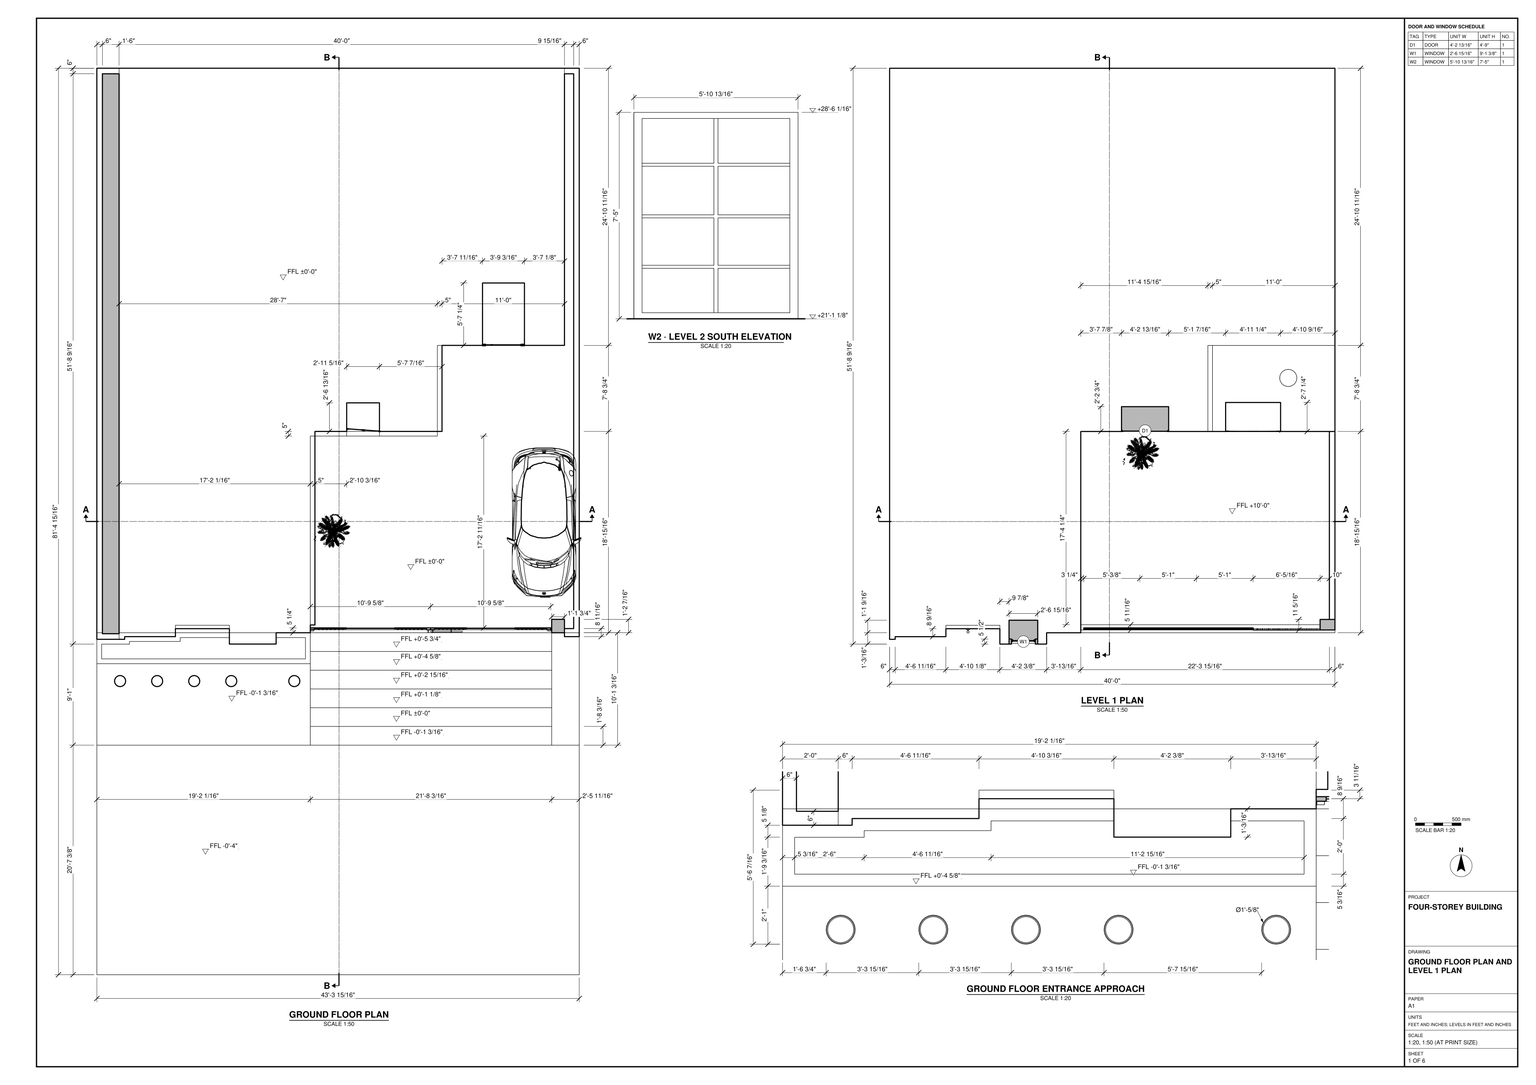
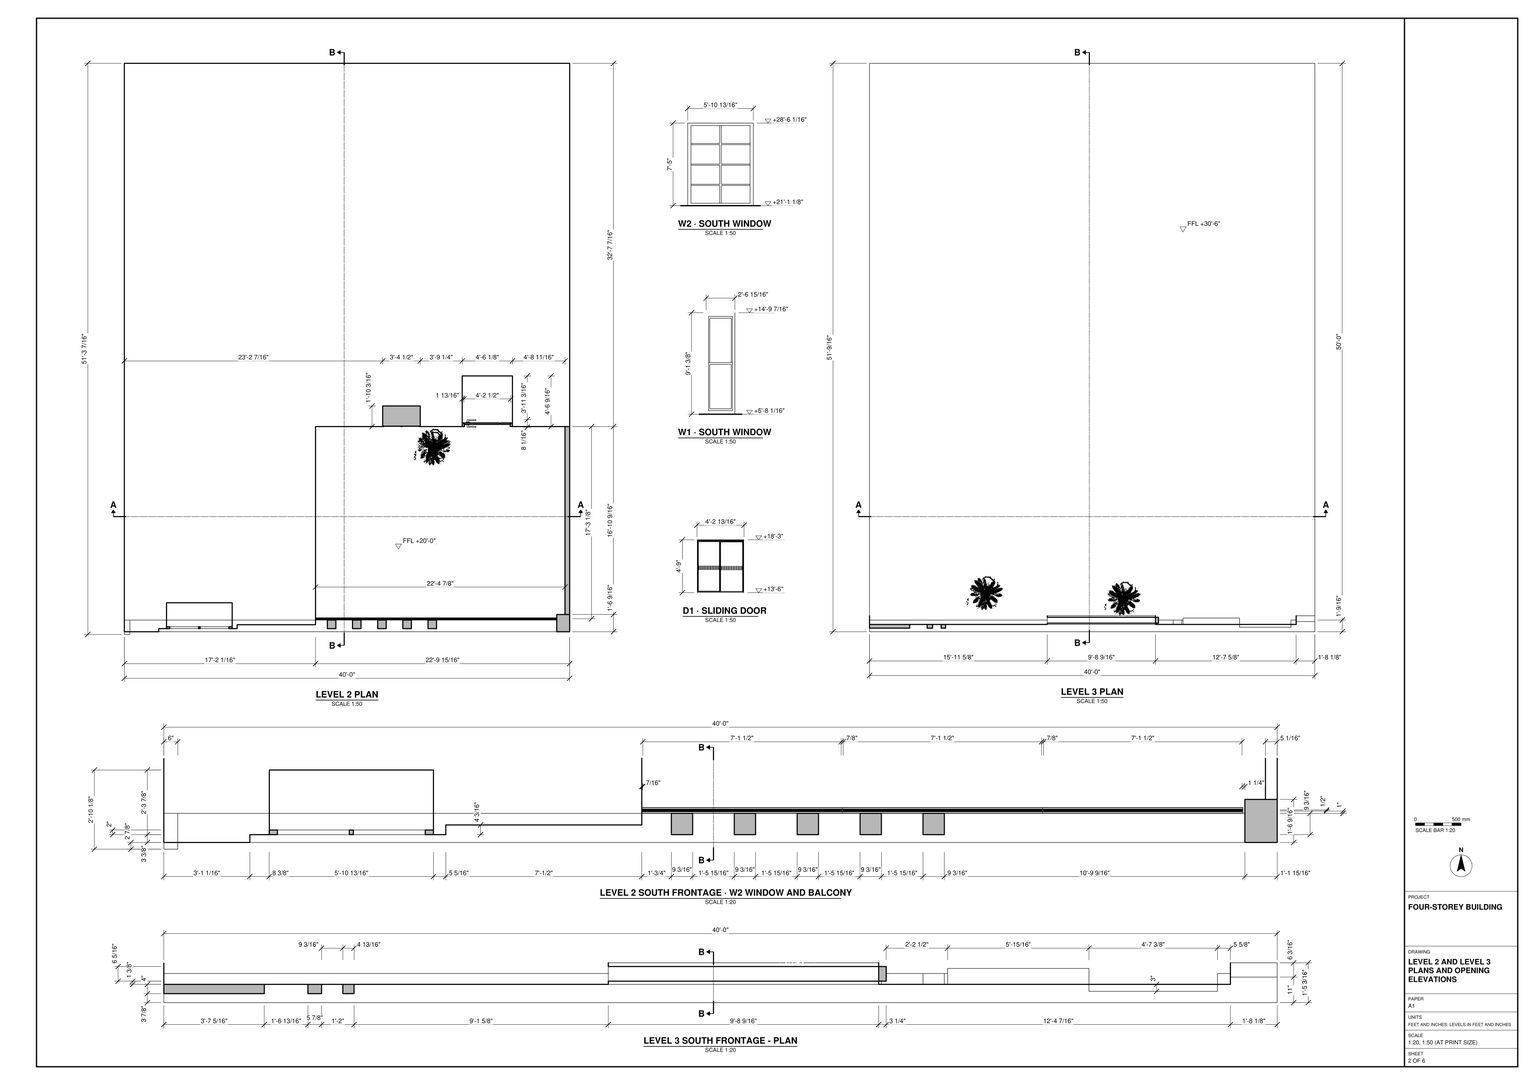
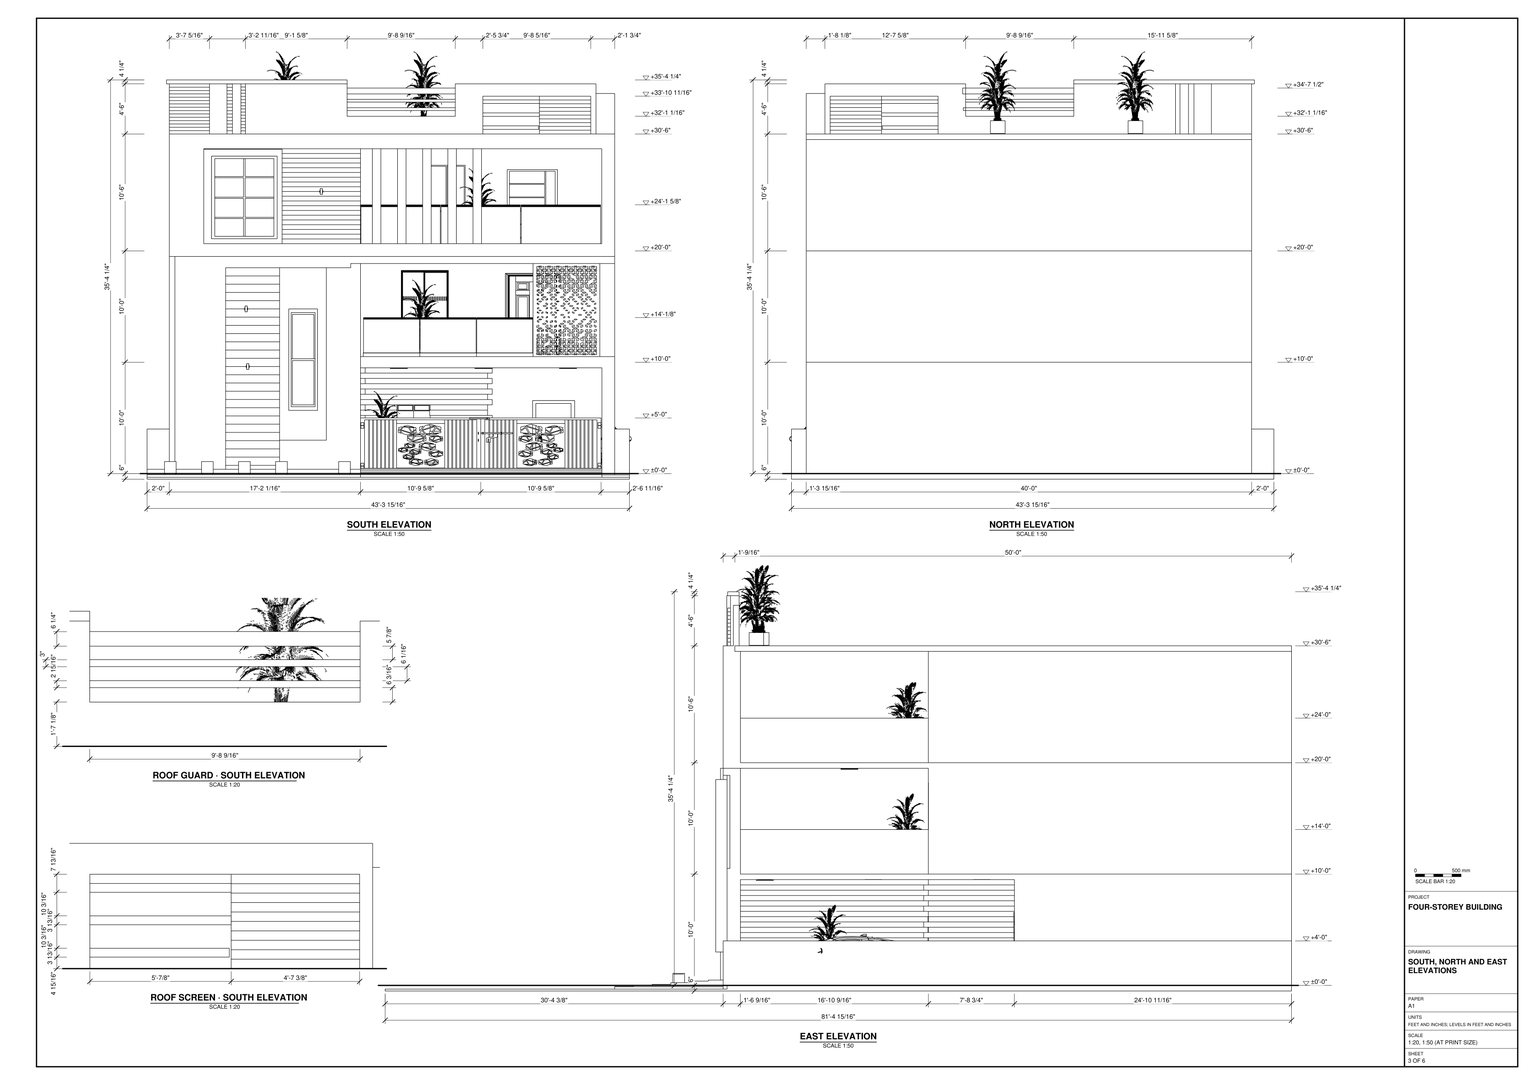
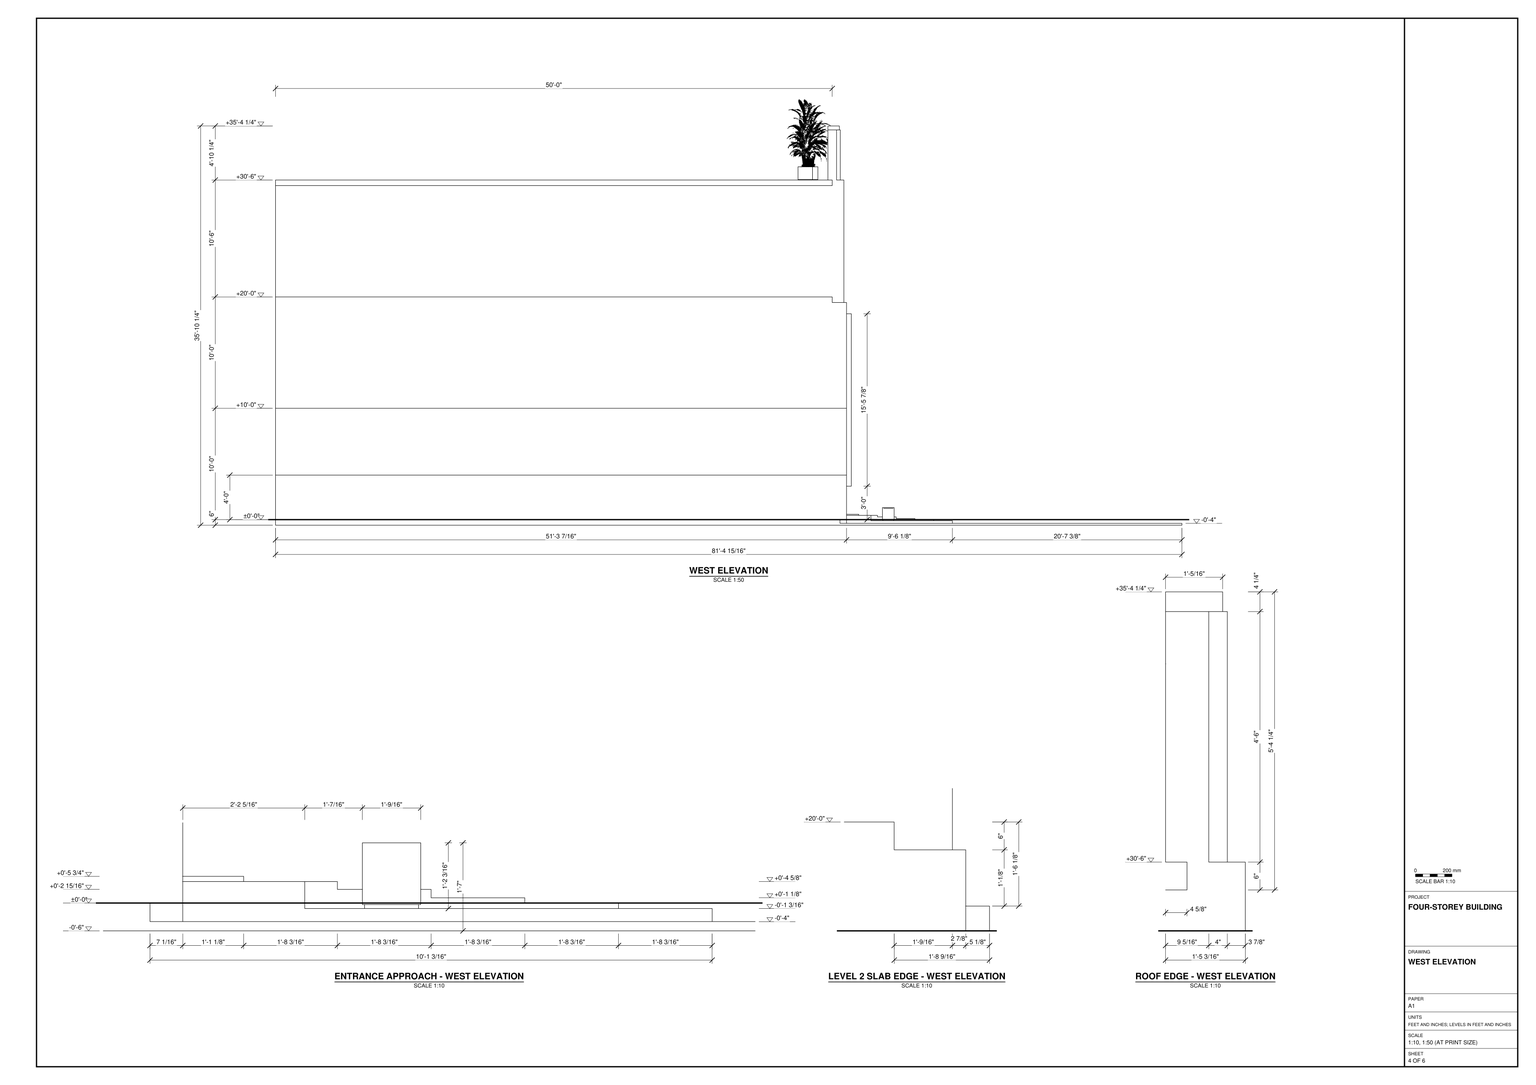
Use task_files/diagram_01.pdf to build the building and its south entrance approach in SketchUp. Work in feet and inches. Including the approach and roof planting, the overall model extents are 43'-5 15/16" across the frontage, 81'-4 15/16" from front to back and 38'-5 9/16" in height. Set the ground floor at ±0'-0", Level 1 at +10'-0", Level 2 at +20'-0" and the roof terrace at +30'-6".

Follow the plans for the wall thicknesses, slab edges and changes in footprint. Set the covered parking bay behind the paired entrance gate on the right when viewed from the south. Model the shallow changes of level across the approach and the two recessed balconies above the bay. Use the opening details for the sliding door, the tall narrow window and the wider divided window. Match the south elevation's projecting window surround, horizontal bands, vertical fins, balcony guards and patterned screen. Finish the flat roof with the stepped parapet, railings and screen shown along its south edge.

Include the parked car and planting in the positions shown. Decor and loose items, including plants and lights, may be any suitable library components. Keep walls, slabs and roof elements in separate groups or components, do the same for each furniture or joinery piece, and use components for repeated parts. Save one SketchUp model as output_files/four_storey_building_with_balconies_and_roof_terrace.skp.

# SketchUp Ruby script. Lengths in inches.
U = 1.inch
M = Sketchup.active_model
def pt(a) = Geom::Point3d.new(a.map { |v| v * U })
def face(e, loops, mat)
  f = e.add_face(loops[0].map { |a| pt(a) })
  loops[1..].each { |l| e.add_face(l.map { |a| pt(a) }).erase! }
  f.material = f.back_material = mat if mat
  f
end
# faces: each face lists its corners as indices into pts; further lists are holes
def faces(e, pts, list, mat = nil) = list.each { |f| face(e, (f[0].is_a?(Array) ? f : [f]).map { |l| l.map { |i| pts[i] } }, mat) }
# xy, xz, yz: faces in a plane at the given z, y or x. An outline is a flat list of corners, or four numbers for a rectangle; further outlines are holes
def ring(l) = l.size == 4 ? [[l[0], l[1]], [l[2], l[1]], [l[2], l[3]], [l[0], l[3]]] : l.each_slice(2).to_a
def flat(e, list, mat, &to3) = list.each { |f| face(e, (f[0].is_a?(Array) ? f : [f]).map { |l| ring(l).map { |u, v| to3.(u, v) } }, mat) }
def xy(e, z, list, mat = nil) = flat(e, list, mat) { |x, y| [x, y, z] }
def xz(e, y, list, mat = nil) = flat(e, list, mat) { |x, z| [x, y, z] }
def yz(e, x, list, mat = nil) = flat(e, list, mat) { |y, z| [x, y, z] }
def lines(e, pts, list) = list.each { |a, b| e.add_line(pt(pts[a]), pt(pts[b])) }
# prism: a flat outline (further loops are holes) pulled along v
def prism(e, loops, v, mat = nil)
  f = face(e, loops, mat); d = Geom::Vector3d.new(v.map { |x| x * U })
  f.pushpull(f.normal.samedirection?(d) ? d.length : -d.length)
end
def box(e, o, s, mat = nil) = prism(e, [[o, [o[0] + s[0], o[1], o[2]], [o[0] + s[0], o[1] + s[1], o[2]], [o[0], o[1] + s[1], o[2]]]], [0, 0, s[2]], mat)
def at(x, y, z, deg = 0) = Geom::Transformation.translation(pt([x, y, z])) * Geom::Transformation.rotation(ORIGIN, Z_AXIS, deg.degrees)
def axes(o, x, y, z) = Geom::Transformation.new([*x, 0, *y, 0, *z, 0, *pt(o).to_a, 1])
def part(name) = M.definitions.add(name)
# library, detail: a bought-in or finely detailed component or shape, given as its bounding box
def library(name, o, s) = part(name).tap { |d| box(d.entities, o, s) }
def detail(e, o, s) = box(e.add_group.entities, o, s)
def put(e, d, t, mat = nil) = e.add_instance(d, t).tap { |i| i.material = mat if mat }
def group(e, t, mat = nil) = e.add_group.tap { |g| g.transformation = t; g.material = mat if mat }.entities
root = M.entities
M.materials.add("2").color = [128, 128, 128]
M.materials["2"].alpha = 0.5
M.materials.add("[0131_Silver]").color = [192, 192, 192]
M.materials.add("[0134_DimGray]").color = [105, 105, 105]
M.materials.add("[0136_Charcoal]").color = [73, 73, 73]
M.materials.add("[0137_Black]").color = [0, 0, 0]
M.materials.add("[Color M00]").color = [255, 255, 255]
M.materials.add("[Color M05]").color = [114, 114, 114]
M.materials.add("[Marble Carrara Floor Tile]").color = [204, 208, 219]
M.materials.add("[Slate Light Tile]").color = [53, 53, 53]
M.materials.add("[Wood Bamboo]").color = [177, 105, 43]
M.materials.add("[Wood Cherry Original]").color = [152, 86, 42]
M.materials.add("[Wood Veneer 01]").color = [120, 70, 37]
c1 = library("jali pattern 2",[0,0,0],[57.36,2,116.36])
c2 = library("Wagner Glass Railing",[9.08,102.375,1.53],[2.51,145.5,42.05])
c3 = library("sliding door",[-94.49,0,0],[94.49,5.91,82.68])
c4 = library("porta 4",[0.2,-5.42,1.33],[46.55,4.72,83.21])
c5 = library("Window 06",[0,0,0],[24,5.5,55])
c6 = library("modern black window",[0,-2,0],[40,2,68])
c7 = library("Glazed double door",[0,0,0],[5.31,78.43,99.16])
c8 = library("PINTU 6 YA",[0,-0.6875,0],[35.83,8.07,80.71])
c9 = part("WindowDoubleBlack")
xy(c9.entities,0,[[0,0,96.0625,1.57]],"[0137_Black]")
xy(c9.entities,2.71,[[2.71,0,46.85,1.57],[49.41,0,93.35,1.57]],"[0137_Black]")
xy(c9.entities,122.09,[[2.71,0,46.85,1.57],[49.41,0,50,1.57],[50,0,93.35,1.57]],"[0137_Black]")
xy(c9.entities,124.8,[[0,0,96.0625,1.57]],"[0137_Black]")
xz(c9.entities,0,[[[0,0,96.0625,124.8],[2.71,2.71,46.85,122.09],[49.41,2.71,93.35,122.09]]],"[0137_Black]")
xz(c9.entities,1.57,[[2.71,2.71,46.85,122.09],[49.41,2.71,93.35,122.09]],"2")
xz(c9.entities,1.57,[[[0,0,96.0625,124.8],[2.71,2.71,46.85,122.09],[49.41,2.71,93.35,122.09]]],"[0137_Black]")
yz(c9.entities,0,[[0,0,1.57,124.8]],"[0137_Black]")
yz(c9.entities,2.71,[[0,2.71,1.57,122.09]],"[0137_Black]")
yz(c9.entities,46.85,[[0,2.71,1.57,122.09]],"[0137_Black]")
yz(c9.entities,49.41,[[0,2.71,1.57,122.09]],"[0137_Black]")
yz(c9.entities,93.35,[[0,2.71,1.57,122.09]],"[0137_Black]")
yz(c9.entities,96.0625,[[0,0,1.57,124.8]],"[0137_Black]")
c10 = library("doors2",[0,0,0],[35.98,7.47,80.98])
c11 = library("Gate_Lasercut_10ftx6ft_Kalil",[-0.15,-3.25,-0.15],[120,5.625,60.3])
c12 = library("Plant",[0,0,0],[12.59,12.59,14.16])
c13 = library("plant\#1",[-22.43,-22.29,0],[44.86,44.58,89.56])
c14 = library("Untitled",[-3.82,8.01,0.375],[80.04,161.09,54.88])
c15 = library("Lamp Wall Outdoor 94-02",[-1.89,-4.65,-3.17],[3.78,4.65,6.35])
c16 = library("Tlon Light 1950 Ceiling 152 010",[-38.39,-38.39,-3.78],[76.78,76.78,3.41])
c17 = library("Dome Light",[-12,-12,0],[24,24,12])
xy(root,-6,[[0,0,519.9375,976.9375]])
xy(root,-4,[[0,247.375,230.0625,247.375,230.0625,368.5625,84.6875,368.5625,84.6875,364.375,30,364.375,30,361.5,0,361.5],[490.25,247.375,519.9375,247.375,519.9375,364.375,504,364.375,504,368.5625,490.25,368.5625],[0,361.5,0,368.5625,84.6875,368.5625,84.6875,364.375,30,364.375,30,361.5],[504,364.375,519.9375,368.5625],[84.6875,368.5625,142.86,372.9375]])
xy(root,-4,[[0,0,519.9375,247.375]],"[Slate Light Tile]")
xy(root,-1.4375,[[490.25,247.375,519.9375,247.375,519.9375,364.375,504,364.375,504,368.5625,490.25,368.5625]],"[Marble Carrara Floor Tile]")
xy(root,-1.1875,[[5.21,340.4,224.86,340.4,224.86,363.36,89.89,363.36,89.89,359.17,35.21,359.17,35.21,356.29,5.21,356.29]])
xy(root,-1.1875,[[0,247.375,230.0625,335.2],[230.0625,247.375,490.25,267.57]],"[Marble Carrara Floor Tile]")
xy(root,0,[[0,361.5,24,361.5,24,367.5,6,367.5,6,368.5625,0,368.5625],[24,361.5,30,361.5,30,364.375,84.6875,364.375,84.6875,368.5625,24,368.5625],[504,364.375,519.9375,368.5625],[6,367.5,24,368.5625],[0,368.5625,0,976.9375,24,976.9375,24,970.9375,6,970.9375,6,368.5625],
  [6,368.5625,24,970.9375],[24,368.5625,84.6875,368.5625,84.6875,372.9375,142.86,372.9375,142.86,368.5625,230.0625,368.5625,230.0625,376.9375,235.0625,376.9375,235.0625,585.5,372.03,585.5,372.03,678.25,415.7,678.25,415.7,745.5,460.89,745.5,460.89,678.25,504,678.25,504,976.9375,24,976.9375],[230.0625,368.5625,490.25,368.5625,490.25,383,504,383,504,373.04,513.9375,373.04,513.9375,970.9375,504,970.9375,504,678.25,460.89,678.25,460.89,745.5,415.7,745.5,415.7,678.25,372.03,678.25,372.03,585.5,235.0625,585.5,235.0625,376.9375,230.0625,376.9375],[504,368.5625,504,373.04,513.9375,373.04,513.9375,970.9375,504,970.9375,504,976.9375,519.9375,976.9375,519.9375,368.5625]])
xy(root,0,[[230.0625,267.57,490.25,287.77]],"[Marble Carrara Floor Tile]")
xy(root,1.125,[[230.0625,287.77,490.25,307.97]],"[Marble Carrara Floor Tile]")
xy(root,2.9375,[[230.0625,307.97,490.25,328.17]],"[Marble Carrara Floor Tile]")
xy(root,4.625,[[[0,335.2,230.0625,335.2,230.0625,368.5625,84.6875,368.5625,84.6875,364.375,30,364.375,30,361.5,0,361.5],[5.21,340.4,5.21,356.29,35.21,356.29,35.21,359.17,89.89,359.17,89.89,363.36,224.86,363.36,224.86,340.4]]])
xy(root,4.625,[[230.0625,328.17,490.25,348.36]],"[Marble Carrara Floor Tile]")
xy(root,5.7,[[230.0625,376.9375,235.0625,580.5],[235.0625,580.5,367.03,585.5],[367.03,585.5,372.03,678.25]],"[Wood Bamboo]")
xy(root,5.75,[[230.0625,348.36,490.25,368.5625]],"[Marble Carrara Floor Tile]")
xy(root,11.4,[[230.0625,376.9375,235.0625,580.5],[235.0625,580.5,367.03,585.5],[367.03,585.5,372.03,678.25]],"[Wood Bamboo]")
xy(root,17.1,[[230.0625,376.9375,235.0625,580.5],[235.0625,580.5,367.03,585.5],[367.03,585.5,372.03,678.25]],"[Wood Bamboo]")
xy(root,22.8,[[230.0625,376.9375,235.0625,580.5],[235.0625,580.5,367.03,585.5],[367.03,585.5,372.03,678.25]],"[Wood Bamboo]")
xy(root,28.5,[[230.0625,376.9375,235.0625,580.5],[235.0625,580.5,367.03,585.5],[367.03,585.5,372.03,678.25]],"[Wood Bamboo]")
xy(root,34.2,[[230.0625,376.9375,235.0625,580.5],[235.0625,580.5,367.03,585.5],[367.03,585.5,372.03,678.25]],"[Wood Bamboo]")
xy(root,36,[[142.86,356.375,193.23,368.5625]])
xy(root,39.9,[[230.0625,376.9375,235.0625,580.5],[235.0625,580.5,269.27,585.5],[304.61,580.5,367.03,585.5],[269.27,585.5,304.61,616.3125],[367.03,585.5,372.03,678.25]],"[Wood Bamboo]")
xy(root,44.375,[[84.6875,372.9375,142.86,376.64]])
xy(root,45.6,[[230.0625,376.9375,235.0625,580.5],[235.0625,580.5,269.27,585.5],[304.61,580.5,367.03,585.5],[367.03,585.5,372.03,678.25]],"[Wood Bamboo]")
xy(root,48,[[0,361.5,24,361.5,24,367.5,6,367.5,6,970.9375,24,970.9375,24,976.9375,0,976.9375],[504,364.375,519.9375,364.375,519.9375,976.9375,504,976.9375,504,970.9375,513.9375,970.9375,513.9375,373.04,504,373.04]])
xy(root,51.3,[[230.0625,376.9375,235.0625,580.5],[235.0625,580.5,269.27,585.5],[304.61,580.5,367.03,585.5],[367.03,585.5,372.03,678.25]],"[Wood Bamboo]")
xy(root,53.25,[[84.6875,372.9375,142.86,376.64]])
xy(root,57,[[230.0625,376.9375,235.0625,580.5],[235.0625,580.5,269.27,585.5],[304.61,580.5,367.03,585.5],[367.03,585.5,372.03,678.25]],"[Wood Bamboo]")
xy(root,62.125,[[84.6875,372.9375,142.86,376.64]])
xy(root,62.7,[[230.0625,376.9375,235.0625,580.5],[235.0625,580.5,269.27,585.5],[304.61,580.5,367.03,585.5],[367.03,585.5,372.03,678.25]],"[Wood Bamboo]")
xy(root,68.09,[[152.74,356.375,183.68,382.125]])
xy(root,68.4,[[230.0625,376.9375,235.0625,580.5],[235.0625,580.5,269.27,585.5],[304.61,580.5,367.03,585.5]],"[Wood Bamboo]")
xy(root,71,[[84.6875,372.9375,142.86,376.64]])
xy(root,74.1,[[230.0625,376.9375,235.0625,585.5],[269.27,585.5,304.61,616.3125],[367.03,585.5,372.03,678.25]],"[Wood Bamboo]")
xy(root,78.75,[[415.7,678.25,460.89,745.5]])
xy(root,79.8,[[230.0625,580.5,367.03,585.5],[367.03,585.5,372.03,678.25]],"[Wood Bamboo]")
xy(root,79.875,[[84.6875,372.9375,142.86,376.64]])
xy(root,85.5,[[230.0625,376.9375,235.0625,580.5],[235.0625,580.5,367.03,585.5],[367.03,585.5,372.03,678.25]],"[Wood Bamboo]")
xy(root,88.75,[[84.6875,372.9375,142.86,376.64]])
xy(root,91.2,[[230.0625,376.9375,235.0625,580.5],[235.0625,580.5,367.03,585.5],[367.03,585.5,372.03,678.25]],"[Wood Bamboo]")
xy(root,96.9,[[230.0625,376.9375,235.0625,580.5],[235.0625,580.5,367.03,585.5],[367.03,585.5,372.03,678.25]],"[Wood Bamboo]")
xy(root,97.625,[[84.6875,372.9375,142.86,376.64]])
xy(root,102.6,[[230.0625,376.9375,235.0625,580.5],[235.0625,580.5,367.03,585.5],[367.03,585.5,372.03,678.25]],"[Wood Bamboo]")
xy(root,106.5,[[84.6875,372.9375,142.86,376.64]])
xy(root,108.3,[[230.0625,376.9375,235.0625,580.5],[235.0625,580.5,367.03,585.5],[367.03,585.5,372.03,678.25]],"[Wood Bamboo]")
xy(root,114,[[230.0625,368.5625,230.0625,376.9375,235.0625,376.9375,235.0625,585.5,372.03,585.5,372.03,678.25,504,678.25,504,383,490.25,383,490.25,368.5625]])
xy(root,115.375,[[84.6875,372.9375,142.86,376.64]])
xy(root,120,[[230.0625,377.28,488,377.28,488,382.9375,498,382.9375,498,585.5,445.42,585.5,445.42,616.75,386.17,616.75,386.17,585.5,230.0625,585.5],[498,382.9375,504,585.5]])
xy(root,123.1875,[[230.0625,371.625,488,377.28]])
xy(root,124.25,[[84.6875,372.9375,142.86,376.64]])
xy(root,126.0625,[[230.0625,368.5625,504,371.625]])
xy(root,133.125,[[84.6875,372.9375,142.86,376.64]])
xy(root,142,[[84.6875,372.9375,142.86,376.64]])
xy(root,150.875,[[84.6875,372.9375,142.86,376.64]])
xy(root,159.75,[[84.6875,372.9375,142.86,376.64]])
xy(root,162.01,[[273.95,585.5,324.76,612.25]])
xy(root,168,[[498,382.9375,504,585.5]])
xy(root,168.625,[[84.6875,372.9375,142.86,376.64]])
xy(root,177.47,[[152.74,356.375,183.68,382.125]])
xy(root,177.5,[[84.6875,372.54,142.86,372.9375],[84.6875,372.9375,142.86,376.64]])
xy(root,186.375,[[84.6875,372.54,142.86,376.64]])
xy(root,195.25,[[84.6875,372.54,142.86,376.64]])
xy(root,204.125,[[84.6875,372.54,142.86,376.64]])
xy(root,213,[[84.6875,372.54,142.86,376.64]])
xy(root,215.87,[[386.17,585.5,445.42,616.75]])
xy(root,219.01,[[273.95,585.5,324.76,612.25]])
xy(root,221.875,[[142.86,356.375,193.23,364.375]])
xy(root,221.875,[[193.23,364.375,219.5,368.5625]],"[Color M05]")
xy(root,221.875,[[84.6875,364.375,142.86,372.54]],"[Wood Bamboo]")
xy(root,226.4,[[219.5,364.375,219.5,368.5625,230.0625,368.5625,230.0625,382.9375,488,382.9375,488,371.625,504,371.625,504,364.375]])
xy(root,234,[[24,361.5,30,364.375],[24,364.375,30,376.9375],[30,364.375,504,376.9375]])
xy(root,234,[[230.0625,382.9375,504,585.5]],"[Color M00]")
xy(root,240,[[24,376.9375,24,976.9375,504,976.9375,504,585.5,442.29,585.5,442.29,640.0625,388.17,640.0625,388.17,585.5,230.0625,585.5,230.0625,376.9375],[230.0625,376.9375,490.07,376.9375,490.07,382.9375,498.9375,382.9375,498.9375,585.5,442.29,585.5,442.29,640.0625,388.17,640.0625,388.17,585.5,230.0625,585.5],[498.9375,382.9375,504,585.5]])
xy(root,247.76,[[61.08,364.375,490.07,364.375,490.07,376.9375,360.49,376.9375,360.49,367.75,351.3,367.75,351.3,376.9375,333.37,376.9375,333.37,367.75,324.18,367.75,324.18,376.9375,306.24,376.9375,306.24,367.75,297.05,367.75,297.05,376.9375,279.12,376.9375,279.12,367.75,269.93,367.75,269.93,376.9375,251.99,376.9375,251.99,367.75,242.8,367.75,242.8,376.9375,230.0625,376.9375,230.0625,371.9375,145.57,371.9375,145.57,367.75,61.08,367.75]])
xy(root,253.1,[[69.49,367.75,140.24,395.625]],"[0131_Silver]")
xy(root,282.27,[[302.44,585.5,342.94,607.6875]])
xy(root,288,[[498.9375,382.9375,504,585.5]])
xy(root,327.58,[[388.17,585.5,442.29,640.0625]])
xy(root,332.27,[[302.44,585.5,342.94,607.6875]])
xy(root,342.13,[[69.49,367.75,140.24,395.625]])
xy(root,349.53,[[61.08,367.75,145.57,371.9375]])
xy(root,350.07,[[[61.08,364.375,61.08,371.9375,230.0625,371.9375,230.0625,382.9375,490.07,382.9375,490.07,364.375],[269.93,367.75,279.12,376.9375],[297.05,367.75,306.24,376.9375]]])
xy(root,350.83,[[351.3,367.75,360.49,376.9375]])
xy(root,351.01,[[324.18,367.75,333.37,376.9375]])
xy(root,356.39,[[242.8,367.75,251.99,376.9375]])
xy(root,360,[[24,376.9375,24,976.9375,504,976.9375,504,585.5,230.0625,585.5,230.0625,382.9375,504,382.9375,504,376.9375],[230.0625,382.9375,504,585.5]])
xy(root,366,[[24,364.375,504,364.375,504,375.375,483.85,375.375,483.85,372.25,478.24,372.25,478.24,376.9375,504,376.9375,504,976.9375,24,976.9375,24,376.9375,361.92,376.9375,361.92,372.25,106,372.25,106,368.25,101.1875,368.25,101.1875,372.25,92,372.25,92,368.25,86.125,368.25,86.125,372.25,67.3125,372.25,67.3125,368.25,24,368.25],[24,368.25,67.3125,372.25],[86.125,368.25,92,372.25],[101.1875,368.25,106,372.25],[422.85,369.25,478.24,372.25]])
xy(root,370.95,[[361.92,374.04,422.05,377.86]],"[0134_DimGray]")
xy(root,374.77,[[361.92,374.04,422.05,377.86]],"[0134_DimGray]")
xy(root,384.92,[[361.92,374.04,422.86,377.86]],"[0134_DimGray]")
xy(root,385.0625,[[215.61,372.25,332.19,381.5625]],"[0134_DimGray]")
xy(root,388.74,[[361.92,374.04,422.86,377.86]],"[0134_DimGray]")
xy(root,391.29,[[215.61,375.125,334.74,378.8125]])
xy(root,394.29,[[215.61,375.125,334.74,378.8125]],"[0134_DimGray]")
xy(root,398.89,[[361.92,374.04,422.85,377.86]],"[0134_DimGray]")
xy(root,400.36,[[215.61,375.125,332.19,378.8125]])
xy(root,402.7,[[361.92,374.04,422.85,377.86]],"[0134_DimGray]")
xy(root,403.36,[[215.61,375.125,332.19,378.8125]],"[0134_DimGray]")
xy(root,406.6875,[[361.92,372.25,422.85,379.125]],"[0134_DimGray]")
xy(root,406.6875,[[422.85,369.25,478.24,372.25]],"[Wood Veneer 01]")
xy(root,409.16,[[215.61,373.63,335.43,379.94]])
xy(root,409.625,[[483.85,375.375,504,381.5625]],"[0134_DimGray]")
xy(root,415.47,[[215.61,373.63,335.43,379.94]],"[0134_DimGray]")
xy(root,420,[[24,368.25,67.3125,369.25],[86.125,368.25,92,369.25],[101.1875,368.25,106,369.25],[24,369.25,67.3125,372.25],[67.3125,369.25,86.125,372.25],
  [86.125,369.25,92,372.25],[92,369.25,101.1875,372.25],[101.1875,369.25,106,372.25],[106,369.25,215.61,372.25],[24,372.25,215.61,381.5625],
  [332.19,372.25,483.85,381.5625]])
xy(root,420,[[21,369.25,24,372.25],[21,372.25,24,381.5625]],"[0134_DimGray]")
xy(root,424.25,[[21,369.25,215.61,381.5625]],"[0134_DimGray]")
xz(root,0,[[0,-6,519.9375,-4]])
xz(root,247.375,[[0,-4,230.0625,-1.1875],[230.0625,-4,490.25,-1.1875],[490.25,-4,519.9375,-1.4375]],"[Marble Carrara Floor Tile]")
xz(root,267.57,[[230.0625,-1.1875,490.25,0]],"[Marble Carrara Floor Tile]")
xz(root,287.77,[[230.0625,0,490.25,1.125]],"[Marble Carrara Floor Tile]")
xz(root,307.97,[[230.0625,1.125,490.25,2.9375]],"[Marble Carrara Floor Tile]")
xz(root,328.17,[[230.0625,2.9375,490.25,4.625]],"[Marble Carrara Floor Tile]")
xz(root,335.2,[[0,-1.1875,230.0625,4.625]])
xz(root,340.4,[[5.21,-1.1875,224.86,4.625]],"[Marble Carrara Floor Tile]")
xz(root,348.36,[[230.0625,4.625,490.25,5.75]],"[Marble Carrara Floor Tile]")
xz(root,356.29,[[5.21,-1.1875,35.21,4.625]])
xz(root,356.375,[[[142.86,36,193.23,221.875],[152.74,68.09,183.68,177.47]]])
xz(root,359.17,[[35.21,-1.1875,89.89,4.625]])
xz(root,361.5,[[0,-4,24,0],[24,-4,30,0],[0,4.625,24,48]])
xz(root,361.5,[[24,4.625,30,234]],"[Color M05]")
xz(root,361.5,[[0,0,24,4.625],[24,0,30,4.625]],"[Marble Carrara Floor Tile]")
xz(root,363.36,[[89.89,-1.1875,142.86,4.625],[142.86,-1.1875,224.86,4.625]])
xz(root,364.375,[[30,-4,84.6875,0],[504,-4,519.9375,-1.4375],[504,-1.4375,519.9375,0],[504,0,519.9375,48],[[24,234,504,366],[61.08,247.76,490.07,350.07]]])
xz(root,364.375,[[30,4.625,84.6875,4.625,84.6875,221.875,219.5,221.875,219.5,226.4,504,226.4,504,234,30,234]],"[Color M05]")
xz(root,364.375,[[30,0,84.6875,4.625]],"[Marble Carrara Floor Tile]")
xz(root,367.5,[[6,0,24,48]])
xz(root,367.75,[[[61.08,247.76,145.57,349.53],[69.49,253.1,140.24,342.13]]],"[0131_Silver]")
xz(root,367.75,[[242.8,247.76,251.99,356.39],[269.93,247.76,279.12,350.07],[297.05,247.76,306.24,350.07],[324.18,247.76,333.37,351.01],[351.3,247.76,360.49,350.83]],"[0136_Charcoal]")
xz(root,368.25,[[86.125,419.85,92,420]])
xz(root,368.25,[[24,366,67.3125,369.6],[86.125,366,92,369.59],[101.1875,366,106,369.375],[101.1875,369.375,106,372.75],[86.125,369.59,92,373.18],
  [24,369.6,67.3125,373.2],[101.1875,372.75,106,376.125],[86.125,373.18,92,376.77],[24,373.2,67.3125,376.8],[101.1875,376.125,106,379.5],
  [86.125,376.77,92,380.36],[24,376.8,67.3125,380.4],[101.1875,379.5,106,382.875],[86.125,380.36,92,383.95],[24,380.4,67.3125,384],
  [101.1875,382.875,106,386.25],[86.125,383.95,92,387.54],[24,384,67.3125,387.6],[101.1875,386.25,106,389.625],[86.125,387.54,92,391.13],
  [24,387.6,67.3125,391.2],[101.1875,389.625,106,393],[86.125,391.13,92,394.72],[24,391.2,67.3125,394.8],[101.1875,393,106,396.375],
  [86.125,394.72,92,398.31],[24,394.8,67.3125,398.4],[101.1875,396.375,106,399.75],[86.125,398.31,92,401.9],[24,398.4,67.3125,402],
  [101.1875,399.75,106,403.125],[86.125,401.9,92,405.49],[24,402,67.3125,405.6],[101.1875,403.125,106,406.5],[86.125,405.49,92,409.08],
  [24,405.6,67.3125,409.2],[101.1875,406.5,106,409.875],[86.125,409.08,92,412.67],[24,409.2,67.3125,412.8],[101.1875,409.875,106,413.25],
  [86.125,412.67,92,416.26],[24,412.8,67.3125,416.4],[101.1875,413.25,106,416.625],[86.125,416.26,92,419.85],[24,416.4,67.3125,420],
  [101.1875,416.625,106,420]],"[Wood Cherry Original]")
xz(root,368.5625,[[0,-4,0,0,84.6875,0,84.6875,4.625,142.86,4.625,142.86,-4],[142.86,-4,230.0625,0],[490.25,-4,504,-1.4375],[504,-4,519.9375,0],[490.25,-1.4375,504,-1.4375,504,126.0625,230.0625,126.0625,230.0625,114,490.25,114],
  [230.0625,0,490.25,5.75],[142.86,4.625,230.0625,4.625,230.0625,226.4,219.5,226.4,219.5,221.875,193.23,221.875,193.23,36,142.86,36]])
xz(root,368.5625,[[142.86,0,230.0625,4.625]],"[Marble Carrara Floor Tile]")
xz(root,369.25,[[21,420,215.61,424.25]],"[0134_DimGray]")
xz(root,369.25,[[422.85,366,478.24,370.07],[422.85,370.07,478.24,374.14],[422.85,374.14,478.24,378.21],[422.85,378.21,478.24,382.28],[422.85,382.28,478.24,386.34],
  [422.85,386.34,478.24,390.41],[422.85,390.41,478.24,394.48],[422.85,394.48,478.24,398.55],[422.85,398.55,478.24,402.62],[422.85,402.62,478.24,406.6875]],"[Wood Veneer 01]")
xz(root,371.625,[[230.0625,123.1875,488,126.0625],[488,126.0625,504,226.4]])
xz(root,371.9375,[[145.57,247.76,230.0625,252.88],[145.57,252.88,230.0625,257.99],[145.57,257.99,230.0625,263.11],[145.57,263.11,230.0625,268.22],[145.57,268.22,230.0625,273.34],
  [145.57,273.34,230.0625,278.45],[145.57,278.45,230.0625,283.57],[145.57,283.57,230.0625,288.68],[145.57,288.68,230.0625,293.8],[145.57,293.8,230.0625,298.92],
  [145.57,298.92,230.0625,304.03],[145.57,304.03,230.0625,309.15],[145.57,309.15,230.0625,314.26],[145.57,314.26,230.0625,319.375],[145.57,319.375,230.0625,324.49],
  [145.57,324.49,230.0625,329.61],[145.57,329.61,230.0625,334.72],[145.57,334.72,230.0625,339.84],[145.57,339.84,230.0625,344.95],[145.57,344.95,230.0625,344.95,230.0625,350.07,61.08,350.07,61.08,349.53,145.57,349.53]],"[0134_DimGray]")
xz(root,372.25,[[24,366,67.3125,420],[67.3125,366,86.125,420],[86.125,366,92,420],[92,366,101.1875,420],[101.1875,366,106,420],
  [106,366,361.92,366,361.92,406.6875,478.24,406.6875,478.24,366,483.85,366,483.85,420,332.19,420,332.19,385.0625,215.61,385.0625,215.61,420,106,420]])
xz(root,372.54,[[84.6875,177.5,142.86,186.375],[84.6875,186.375,142.86,195.25],[84.6875,195.25,142.86,204.125],[84.6875,204.125,142.86,213],[84.6875,213,142.86,221.875]],"[Wood Bamboo]")
xz(root,372.9375,[[84.6875,-4,142.86,0]])
xz(root,372.9375,[[84.6875,0,142.86,8.875],[84.6875,8.875,142.86,17.75],[84.6875,17.75,142.86,26.625],[84.6875,26.625,142.86,35.5],[84.6875,35.5,142.86,44.375],
  [84.6875,44.375,142.86,53.25],[84.6875,53.25,142.86,62.125],[84.6875,62.125,142.86,71],[84.6875,71,142.86,79.875],[84.6875,79.875,142.86,88.75],
  [84.6875,88.75,142.86,97.625],[84.6875,97.625,142.86,106.5],[84.6875,106.5,142.86,115.375],[84.6875,115.375,142.86,124.25],[84.6875,124.25,142.86,133.125],
  [84.6875,133.125,142.86,142],[84.6875,142,142.86,150.875],[84.6875,150.875,142.86,159.75],[84.6875,159.75,142.86,168.625],[84.6875,168.625,142.86,177.5]],"[Wood Bamboo]")
xz(root,373.04,[[504,0,513.9375,48]])
xz(root,373.63,[[215.61,409.16,335.43,415.47]],"[0134_DimGray]")
xz(root,374.04,[[361.92,370.95,422.05,374.77],[361.92,384.92,422.86,388.74],[361.92,398.89,422.85,402.7]],"[0134_DimGray]")
xz(root,375.125,[[215.61,391.29,334.74,394.29],[215.61,400.36,332.19,403.36]],"[0134_DimGray]")
xz(root,375.375,[[483.85,366,504,409.625]],"[0134_DimGray]")
xz(root,376.9375,[[24,234,230.0625,240],[230.0625,234,490.07,240],[230.0625,240,230.0625,247.76,242.8,247.76,242.8,356.39,251.99,356.39,251.99,247.76,269.93,247.76,269.93,350.07,279.12,350.07,279.12,247.76,297.05,247.76,297.05,350.07,306.24,350.07,306.24,247.76,324.18,247.76,324.18,351.01,333.37,351.01,333.37,247.76,351.3,247.76,351.3,350.83,360.49,350.83,360.49,247.76,490.07,247.76,490.07,240]])
xz(root,376.9375,[[230.0625,0,235.0625,5.7],[230.0625,11.4,235.0625,17.1],[230.0625,22.8,235.0625,28.5],[230.0625,34.2,235.0625,39.9],[230.0625,45.6,235.0625,51.3],
  [230.0625,57,235.0625,62.7],[230.0625,68.4,235.0625,74.1],[230.0625,85.5,235.0625,91.2],[230.0625,96.9,235.0625,102.6],[230.0625,108.3,235.0625,114]],"[Wood Bamboo]")
xz(root,377.28,[[230.0625,120,488,123.1875]])
xz(root,377.86,[[361.92,370.95,422.05,374.77],[361.92,384.92,422.86,388.74],[361.92,398.89,422.85,402.7]])
xz(root,378.8125,[[215.61,391.29,334.74,394.29],[215.61,400.36,332.19,403.36]])
xz(root,379.94,[[215.61,409.16,335.43,415.47]])
xz(root,381.5625,[[21,420,215.61,424.25]])
xz(root,382.125,[[152.74,68.09,183.68,177.47]])
xz(root,382.9375,[[488,120,488,226.4,230.0625,226.4,230.0625,234,504,234,504,168,498,168,498,120],[498,120,504,168],[490.07,240,490.07,350.07,230.0625,350.07,230.0625,360,504,360,504,288,498.9375,288,498.9375,240],[498.9375,240,504,288]])
xz(root,383,[[490.25,0,504,114]])
xz(root,395.625,[[69.49,253.1,140.24,342.13]],"[0131_Silver]")
xz(root,580.5,[[230.0625,5.7,367.03,11.4],[230.0625,17.1,367.03,22.8],[230.0625,28.5,367.03,34.2],[230.0625,39.9,269.27,45.6],[304.61,39.9,367.03,45.6],
  [230.0625,51.3,269.27,57],[304.61,51.3,367.03,57],[230.0625,62.7,269.27,68.4],[304.61,62.7,367.03,68.4],[230.0625,79.8,367.03,85.5],
  [230.0625,91.2,367.03,96.9],[230.0625,102.6,367.03,108.3]],"[Wood Bamboo]")
xz(root,585.5,[[[230.0625,120,386.17,120,386.17,215.87,445.42,215.87,445.42,120,498,120,498,168,504,168,504,234,230.0625,234],[273.95,162.01,324.76,219.01]],[498,120,504,168],[[230.0625,240,388.17,240,388.17,327.58,442.29,327.58,442.29,240,498.9375,240,498.9375,288,504,288,504,360,230.0625,360],[302.44,282.27,342.94,332.27]],[498.9375,240,504,288]])
xz(root,585.5,[[235.0625,0,372.03,5.7],[235.0625,11.4,372.03,17.1],[235.0625,22.8,372.03,28.5],[235.0625,34.2,372.03,39.9],[235.0625,45.6,269.27,51.3],
  [304.61,45.6,372.03,51.3],[235.0625,57,269.27,62.7],[304.61,57,372.03,62.7],[235.0625,68.4,269.27,74.1],[304.61,68.4,367.03,74.1],
  [230.0625,74.1,372.03,79.8],[235.0625,85.5,372.03,91.2],[235.0625,96.9,372.03,102.6],[235.0625,108.3,372.03,114]],"[Wood Bamboo]")
xz(root,607.6875,[[302.44,282.27,342.94,332.27]])
xz(root,612.25,[[273.95,162.01,324.76,219.01]])
xz(root,616.3125,[[269.27,39.9,304.61,74.1]],"[Wood Bamboo]")
xz(root,616.75,[[386.17,120,445.42,215.87]])
xz(root,640.0625,[[388.17,240,442.29,327.58]])
xz(root,678.25,[[372.03,0,415.7,0,415.7,78.75,460.89,78.75,460.89,0,504,0,504,114,372.03,114,372.03,108.3,367.03,108.3,367.03,102.6,372.03,102.6,372.03,96.9,367.03,96.9,367.03,91.2,372.03,91.2,372.03,85.5,367.03,85.5,367.03,79.8,372.03,79.8,372.03,74.1,367.03,74.1,367.03,62.7,372.03,62.7,372.03,57,367.03,57,367.03,51.3,372.03,51.3,372.03,45.6,367.03,45.6,367.03,39.9,372.03,39.9,372.03,34.2,367.03,34.2,367.03,28.5,372.03,28.5,372.03,22.8,367.03,22.8,367.03,17.1,372.03,17.1,372.03,11.4,367.03,11.4,367.03,5.7,372.03,5.7]])
xz(root,745.5,[[415.7,0,460.89,78.75]])
xz(root,970.9375,[[6,0,24,48],[504,0,513.9375,48]])
xz(root,976.9375,[[0,-6,519.9375,0],[0,0,24,48],[24,0,504,120],[504,0,519.9375,48],[24,120,504,240],
  [24,240,504,360],[24,360,504,366]])
yz(root,0,[[0,-6,0,-4,368.5625,-4,368.5625,0,976.9375,0,976.9375,-6],[247.375,-4,247.375,-1.1875,335.2,-1.1875,335.2,4.625,361.5,4.625,361.5,-4],[361.5,-4,368.5625,0],[361.5,0,976.9375,48]])
yz(root,5.21,[[340.4,-1.1875,356.29,4.625]])
yz(root,6,[[367.5,0,970.9375,48]])
yz(root,21,[[369.25,420,381.5625,424.25]],"[0134_DimGray]")
yz(root,24,[[367.5,0,367.5,48,361.5,48,361.5,120,976.9375,120,976.9375,48,970.9375,48,970.9375,0],[361.5,120,361.5,234,376.9375,234,376.9375,240,976.9375,240,976.9375,120],[364.375,234,364.375,366,372.25,366,372.25,420,381.5625,420,381.5625,366,376.9375,366,376.9375,360,976.9375,360,976.9375,240,376.9375,240,376.9375,234],[376.9375,360,976.9375,366],[368.25,366,372.25,420]])
yz(root,30,[[361.5,-4,364.375,0],[361.5,4.625,364.375,234]])
yz(root,30,[[361.5,0,364.375,4.625]],"[Marble Carrara Floor Tile]")
yz(root,35.21,[[356.29,-1.1875,359.17,4.625]])
yz(root,61.08,[[364.375,247.76,367.75,247.76,367.75,349.53,371.9375,349.53,371.9375,350.07,364.375,350.07]])
yz(root,67.3125,[[368.25,366,372.25,420]],"[Wood Cherry Original]")
yz(root,69.49,[[367.75,253.1,395.625,342.13]],"[0131_Silver]")
yz(root,84.6875,[[364.375,-4,372.9375,0]])
yz(root,84.6875,[[364.375,0,368.5625,4.625]],"[Marble Carrara Floor Tile]")
yz(root,84.6875,[[368.5625,0,372.9375,0,372.9375,177.5,372.54,177.5,372.54,221.875,364.375,221.875,364.375,4.625,368.5625,4.625]],"[Wood Bamboo]")
yz(root,86.125,[[368.25,366,372.25,420]],"[Wood Cherry Original]")
yz(root,89.89,[[359.17,-1.1875,363.36,4.625]])
yz(root,92,[[368.25,366,372.25,420]],"[Wood Cherry Original]")
yz(root,101.1875,[[368.25,366,372.25,420]],"[Wood Cherry Original]")
yz(root,106,[[368.25,366,372.25,420]],"[Wood Cherry Original]")
yz(root,140.24,[[367.75,253.1,395.625,342.13]])
yz(root,142.86,[[368.5625,-4,372.9375,0],[368.5625,0,372.9375,8.875],[368.5625,8.875,372.9375,17.75],[368.5625,17.75,372.9375,26.625],[368.5625,26.625,372.9375,35.5],
  [368.5625,35.5,372.9375,36]])
yz(root,142.86,[[356.375,36,356.375,221.875,372.54,221.875,372.54,177.5,372.9375,177.5,372.9375,36]],"[Wood Bamboo]")
yz(root,145.57,[[367.75,247.76,371.9375,349.53]])
yz(root,152.74,[[356.375,68.09,382.125,177.47]])
yz(root,183.68,[[356.375,68.09,382.125,177.47]])
yz(root,193.23,[[356.375,36,368.5625,221.875]])
yz(root,215.61,[[[372.25,385.0625,381.5625,420],[373.63,409.16,379.94,415.47],[375.125,400.36,378.8125,403.36],[375.125,391.29,378.8125,394.29]],[369.25,420,381.5625,424.25]])
yz(root,219.5,[[364.375,221.875,368.5625,226.4]],"[Color M05]")
yz(root,224.86,[[340.4,-1.1875,363.36,4.625]])
yz(root,230.0625,[[247.375,-4,368.5625,-4,368.5625,4.625,335.2,4.625,335.2,-1.1875,247.375,-1.1875],[377.28,120,585.5,120,585.5,234,382.9375,234,382.9375,226.4,368.5625,226.4,368.5625,126.0625,371.625,126.0625,371.625,123.1875,377.28,123.1875],[368.5625,123.1875,371.625,126.0625],[376.9375,240,585.5,240,585.5,360,382.9375,360,382.9375,350.07,371.9375,350.07,371.9375,247.76,376.9375,247.76]])
yz(root,230.0625,[[368.5625,0,376.9375,114]],"[Color M00]")
yz(root,230.0625,[[267.57,-1.1875,335.2,-1.1875,335.2,4.625,328.17,4.625,328.17,2.9375,307.97,2.9375,307.97,1.125,287.77,1.125,287.77,0,267.57,0],[348.36,4.625,368.5625,5.75]],"[Marble Carrara Floor Tile]")
yz(root,230.0625,[[376.9375,5.7,580.5,11.4],[376.9375,17.1,580.5,22.8],[376.9375,28.5,580.5,34.2],[376.9375,39.9,580.5,45.6],[376.9375,51.3,580.5,57],
  [376.9375,62.7,580.5,68.4],[376.9375,74.1,585.5,79.8],[376.9375,79.8,580.5,85.5],[376.9375,91.2,580.5,96.9],[376.9375,102.6,580.5,108.3]],"[Wood Bamboo]")
yz(root,235.0625,[[376.9375,0,585.5,5.7],[376.9375,11.4,585.5,17.1],[376.9375,22.8,585.5,28.5],[376.9375,34.2,585.5,39.9],[376.9375,45.6,585.5,51.3],
  [376.9375,57,585.5,62.7],[376.9375,68.4,585.5,74.1],[376.9375,85.5,585.5,91.2],[376.9375,96.9,585.5,102.6],[376.9375,108.3,585.5,114]],"[Wood Bamboo]")
yz(root,242.8,[[367.75,247.76,376.9375,356.39]],"[0136_Charcoal]")
yz(root,251.99,[[367.75,247.76,376.9375,356.39]],"[0136_Charcoal]")
yz(root,269.27,[[580.5,39.9,616.3125,39.9,616.3125,74.1,585.5,74.1,585.5,68.4,580.5,68.4,580.5,62.7,585.5,62.7,585.5,57,580.5,57,580.5,51.3,585.5,51.3,585.5,45.6,580.5,45.6]],"[Wood Bamboo]")
yz(root,269.93,[[367.75,247.76,376.9375,350.07]],"[0136_Charcoal]")
yz(root,273.95,[[585.5,162.01,612.25,219.01]])
yz(root,279.12,[[367.75,247.76,376.9375,350.07]],"[0136_Charcoal]")
yz(root,297.05,[[367.75,247.76,376.9375,350.07]],"[0136_Charcoal]")
yz(root,302.44,[[585.5,282.27,607.6875,332.27]])
yz(root,304.61,[[580.5,39.9,580.5,45.6,585.5,45.6,585.5,51.3,580.5,51.3,580.5,57,585.5,57,585.5,62.7,580.5,62.7,580.5,68.4,585.5,68.4,585.5,74.1,616.3125,74.1,616.3125,39.9]],"[Wood Bamboo]")
yz(root,306.24,[[367.75,247.76,376.9375,350.07]],"[0136_Charcoal]")
yz(root,324.18,[[367.75,247.76,376.9375,351.01]],"[0136_Charcoal]")
yz(root,324.76,[[585.5,162.01,612.25,219.01]])
yz(root,332.19,[[[372.25,385.0625,381.5625,420],[375.125,400.36,378.8125,403.36]]],"[0134_DimGray]")
yz(root,333.37,[[367.75,247.76,376.9375,351.01]],"[0136_Charcoal]")
yz(root,334.74,[[375.125,391.29,378.8125,394.29]])
yz(root,335.43,[[373.63,409.16,379.94,415.47]])
yz(root,342.94,[[585.5,282.27,607.6875,332.27]])
yz(root,351.3,[[367.75,247.76,376.9375,350.83]],"[0136_Charcoal]")
yz(root,360.49,[[367.75,247.76,376.9375,350.83]],"[0136_Charcoal]")
yz(root,361.92,[[[372.25,366,379.125,406.6875],[374.04,398.89,377.86,402.7],[374.04,384.92,377.86,388.74],[374.04,370.95,377.86,374.77]]],"[0134_DimGray]")
yz(root,367.03,[[580.5,5.7,678.25,11.4],[580.5,17.1,678.25,22.8],[580.5,28.5,678.25,34.2],[580.5,39.9,678.25,45.6],[580.5,51.3,678.25,57],
  [580.5,62.7,678.25,68.4],[585.5,68.4,678.25,74.1],[580.5,79.8,678.25,85.5],[580.5,91.2,678.25,96.9],[580.5,102.6,678.25,108.3]],"[Wood Bamboo]")
yz(root,372.03,[[585.5,0,678.25,5.7],[585.5,11.4,678.25,17.1],[585.5,22.8,678.25,28.5],[585.5,34.2,678.25,39.9],[585.5,45.6,678.25,51.3],
  [585.5,57,678.25,62.7],[585.5,74.1,678.25,79.8],[585.5,85.5,678.25,91.2],[585.5,96.9,678.25,102.6],[585.5,108.3,678.25,114]],"[Wood Bamboo]")
yz(root,386.17,[[585.5,120,616.75,215.87]])
yz(root,388.17,[[585.5,240,640.0625,327.58]])
yz(root,415.7,[[678.25,0,745.5,78.75]])
yz(root,422.05,[[374.04,370.95,377.86,374.77]])
yz(root,422.85,[[[369.25,366,379.125,406.6875],[374.04,398.89,377.86,402.7]]],"[0134_DimGray]")
yz(root,422.86,[[374.04,384.92,377.86,388.74]])
yz(root,442.29,[[585.5,240,640.0625,327.58]])
yz(root,445.42,[[585.5,120,616.75,215.87]])
yz(root,460.89,[[678.25,0,745.5,78.75]])
yz(root,478.24,[[369.25,366,372.25,370.07],[369.25,370.07,372.25,374.14],[369.25,374.14,372.25,378.21],[369.25,378.21,372.25,382.28],[369.25,382.28,372.25,386.34],
  [369.25,386.34,372.25,390.41],[369.25,390.41,372.25,394.48],[369.25,394.48,372.25,398.55],[369.25,398.55,372.25,402.62],[369.25,402.62,372.25,406.6875]],"[Wood Veneer 01]")
yz(root,483.85,[[372.25,366,375.375,366,375.375,409.625,381.5625,409.625,381.5625,420,372.25,420]])
yz(root,488,[[377.28,120,377.28,123.1875,371.625,123.1875,371.625,226.4,382.9375,226.4,382.9375,120]])
yz(root,490.07,[[376.9375,240,376.9375,247.76,364.375,247.76,364.375,350.07,382.9375,350.07,382.9375,240]])
yz(root,490.25,[[247.375,-4,368.5625,-1.4375],[368.5625,0,383,114]])
yz(root,490.25,[[247.375,-1.4375,247.375,-1.1875,267.57,-1.1875,267.57,0,287.77,0,287.77,1.125,307.97,1.125,307.97,2.9375,328.17,2.9375,328.17,4.625,348.36,4.625,348.36,5.75,368.5625,5.75,368.5625,-1.4375]],"[Marble Carrara Floor Tile]")
yz(root,498,[[382.9375,120,585.5,168]])
yz(root,498.9375,[[382.9375,240,585.5,288]])
yz(root,504,[[364.375,-4,368.5625,-1.4375],[364.375,-1.4375,368.5625,0],[364.375,0,368.5625,48],[373.04,0,383,0,383,114,678.25,114,678.25,0,970.9375,0,970.9375,48,976.9375,48,976.9375,120,382.9375,120,382.9375,234,364.375,234,364.375,226.4,371.625,226.4,371.625,126.0625,368.5625,126.0625,368.5625,48,373.04,48],[368.5625,0,373.04,48],
  [382.9375,120,585.5,168],[382.9375,240,585.5,288],[585.5,240,976.9375,360],[376.9375,360,976.9375,366]])
yz(root,504,[[585.5,120,976.9375,120,976.9375,240,382.9375,240,382.9375,360,376.9375,360,376.9375,366,381.5625,366,381.5625,409.625,375.375,409.625,375.375,366,364.375,366,364.375,234,585.5,234]],"[0134_DimGray]")
yz(root,513.9375,[[373.04,0,970.9375,48]])
yz(root,519.9375,[[0,-6,976.9375,-6,976.9375,0,368.5625,0,368.5625,-4,0,-4],[364.375,-4,368.5625,0],[364.375,0,976.9375,48]])
yz(root,519.9375,[[247.375,-4,364.375,-1.4375]],"[Marble Carrara Floor Tile]")
p = [[490.07,376.9375,240],[504,376.9375,240],[64.16,376.9375,344.95],[145.57,376.9375,344.95],[64.16,376.9375,252.88],[145.57,376.9375,252.88],
  [64.16,376.9375,247.76],[145.57,376.9375,247.76],[488,377.28,120],[488,371.625,120]]
lines(root,p,[[0,1],[2,3],[4,5],[6,7],[8,9]])
put(root,c1,axes([416.01,371.625,126.0625],[1.2551,0,0],[0,0.77,0],[0,0,0.8623]))
put(root,c2,axes([104.21,383.22,124.53],[0,-1,0],[1.25788,0,0],[0,0,1]))
put(root,c2,axes([47.6875,388.53,238.19],[0,-1,0],[1.78144,0,0],[0,0,1.18]))
put(root,c3,axes([324.76,585.5,162.01],[0.53777,0,0],[0,0.31,0],[0,0,0.68943]))
put(root,c4,axes([415.38,680.9,-1.27],[0.9734,0,0],[0,0.62,0],[0,0,0.94657]))
put(root,c5,axes([152.74,356.375,68.09],[1.29,0,0],[0,1,0],[0,0,1.98864]))
put(root,c6,axes([69.4375,369.75,253.1],[1.77,0,0],[0,1,0],[0,0,1.30848]))
put(root,c7,axes([305.13,585.08,39.9],[0.01435,0.19547,0],[-0.45514,0.03342,0],[0,0,0.34491]))
put(root,c8,axes([388.17,585.5,240],[1.51,0,0],[0,1,0],[0,0,1.08509]))
put(root,c9,axes([302.44,585.5,282.27],[0.4216,0,0],[0,0.25,0],[0,0,0.40063]))
put(root,c10,axes([386.17,585.8,120],[1.64655,0,0],[0,-0.04008,0],[0,0,1.18379]))
put(root,c11,axes([230.39,371.8125,0.15],[2.16,0,0],[0,1,0],[0,0,1]))
put(root,c12,at(206.52,310.2,-1.1875))
put(root,c12,at(138.58,310.2,-1.1875))
put(root,c12,at(98.65,310.2,-1.1875))
put(root,c12,at(58.71,310.2,-1.1875))
put(root,c12,at(18.77,310.2,-1.1875))
put(root,c13,at(254.625,477.43,0))
put(root,c13,at(296.0625,561.35,120))
put(root,c13,at(356.99,563.91,240))
put(root,c13,at(356.99,560.91,240))
put(root,c13,at(149.25,405.01,366))
put(root,c13,at(297.64,399.23,366))
put(root,c14,at(445.82,398.73,0))
put(root,c15,at(187.82,371.9375,304.03))
put(root,c15,at(106.78,372.54,177.5))
put(root,c15,at(108.52,372.9375,115.375))
put(root,c16,axes([271.53,500.41,233.72],[0.24,0,0],[0,0.24,0],[0,0,0.24]))
put(root,c16,axes([443.4,500.41,233.72],[0.24,0,0],[0,0.24,0],[0,0,0.24]))
put(root,c16,axes([309.43,509.76,360.91],[0.24,0,0],[0,0.24,0],[0,0,0.24]))
put(root,c16,axes([456.37,509.76,360.91],[0.24,0,0],[0,0.24,0],[0,0,0.24]))
put(root,c16,axes([453.68,409.32,114.09],[0.24,0,0],[0,0.24,0],[0,0,0.24]))
put(root,c16,axes([453.68,409.32,114.91],[0.24,0,0],[0,0.24,0],[0,0,0.24]))
put(root,c16,axes([453.68,526.25,114.91],[0.24,0,0],[0,0.24,0],[0,0,0.24]))
put(root,c16,axes([453.68,643.19,114.91],[0.24,0,0],[0,0.24,0],[0,0,0.24]))
put(root,c16,axes([362.53,409.32,114.09],[0.24,0,0],[0,0.24,0],[0,0,0.24]))
put(root,c16,axes([271.37,409.32,114.09],[0.24,0,0],[0,0.24,0],[0,0,0.24]))
put(root,c17,at(-10.78,477.57,0))
